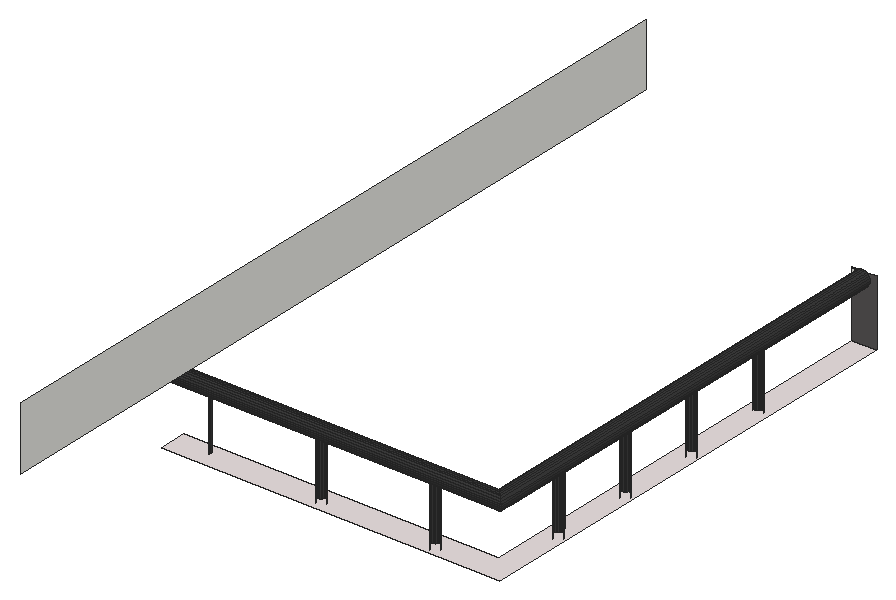
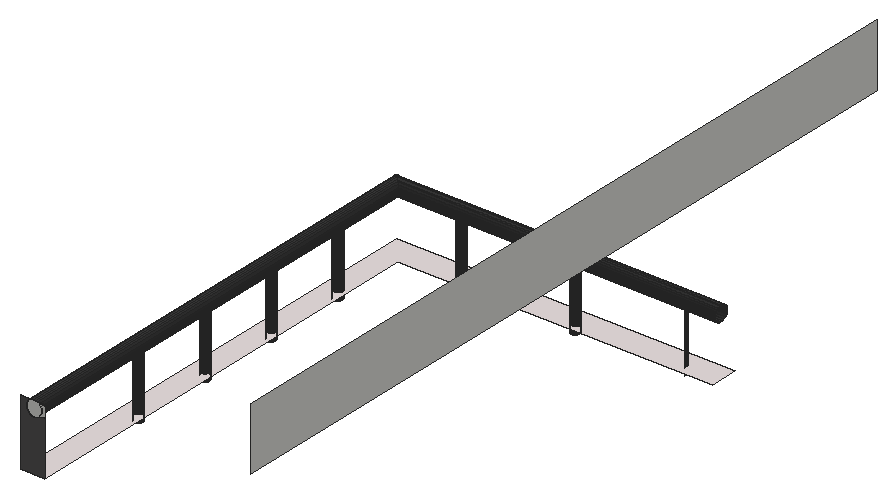
# SketchUp Ruby script. Lengths in inches.
U = 1.inch
M = Sketchup.active_model
def pt(a) = Geom::Point3d.new(a.map { |v| v * U })
def face(e, loops, mat)
  f = e.add_face(loops[0].map { |a| pt(a) })
  loops[1..].each { |l| e.add_face(l.map { |a| pt(a) }).erase! }
  f.material = f.back_material = mat if mat
  f
end
# faces: each face lists its corners as indices into pts; further lists are holes
def faces(e, pts, list, mat = nil) = list.each { |f| face(e, (f[0].is_a?(Array) ? f : [f]).map { |l| l.map { |i| pts[i] } }, mat) }
# xy, xz, yz: faces in a plane at the given z, y or x. An outline is a flat list of corners, or four numbers for a rectangle; further outlines are holes
def ring(l) = l.size == 4 ? [[l[0], l[1]], [l[2], l[1]], [l[2], l[3]], [l[0], l[3]]] : l.each_slice(2).to_a
def flat(e, list, mat, &to3) = list.each { |f| face(e, (f[0].is_a?(Array) ? f : [f]).map { |l| ring(l).map { |u, v| to3.(u, v) } }, mat) }
def xy(e, z, list, mat = nil) = flat(e, list, mat) { |x, y| [x, y, z] }
def xz(e, y, list, mat = nil) = flat(e, list, mat) { |x, z| [x, y, z] }
def yz(e, x, list, mat = nil) = flat(e, list, mat) { |y, z| [x, y, z] }
def lines(e, pts, list) = list.each { |a, b| e.add_line(pt(pts[a]), pt(pts[b])) }
# prism: a flat outline (further loops are holes) pulled along v
def prism(e, loops, v, mat = nil)
  f = face(e, loops, mat); d = Geom::Vector3d.new(v.map { |x| x * U })
  f.pushpull(f.normal.samedirection?(d) ? d.length : -d.length)
end
def box(e, o, s, mat = nil) = prism(e, [[o, [o[0] + s[0], o[1], o[2]], [o[0] + s[0], o[1] + s[1], o[2]], [o[0], o[1] + s[1], o[2]]]], [0, 0, s[2]], mat)
def at(x, y, z, deg = 0) = Geom::Transformation.translation(pt([x, y, z])) * Geom::Transformation.rotation(ORIGIN, Z_AXIS, deg.degrees)
def axes(o, x, y, z) = Geom::Transformation.new([*x, 0, *y, 0, *z, 0, *pt(o).to_a, 1])
def part(name) = M.definitions.add(name)
# library, detail: a bought-in or finely detailed component or shape, given as its bounding box
def library(name, o, s) = part(name).tap { |d| box(d.entities, o, s) }
def detail(e, o, s) = box(e.add_group.entities, o, s)
def put(e, d, t, mat = nil) = e.add_instance(d, t).tap { |i| i.material = mat if mat }
def group(e, t, mat = nil) = e.add_group.tap { |g| g.transformation = t; g.material = mat if mat }.entities
root = M.entities
M.materials.add("Generic\#2").color = [87, 84, 84]
M.materials.add("Generic\#9").color = [233, 223, 223]
M.materials.add("[Color M07]").color = [58, 58, 58]
xy(root,272.4375,[[470.29,127.4375,518.6875,127.4375,518.6875,194.75,515.25,194.75,515.25,131.45,470.29,131.45]],"Generic\#9")
xz(root,194.75,[[516.7,279.83,516.99,279.87,517.26,279.98,517.49,280.16,517.66,280.39,517.77,280.65,517.8125,280.94,517.77,281.23,517.66,281.49,517.49,281.72,517.26,281.9,516.15,281.9,515.9375,281.74,515.25,281.74,515.25,280.14,515.9375,280.14,516.15,279.98,516.42,279.87],[515.25,281.74,515.9375,281.74,516.15,281.9,515.25,281.9]])
xz(root,194.75,[[515.25,272.4375,518.6875,272.4375,518.6875,281.9,517.26,281.9,517.49,281.72,517.66,281.49,517.77,281.23,517.8125,280.94,517.77,280.65,517.66,280.39,517.49,280.16,517.26,279.98,516.99,279.87,516.7,279.83,516.42,279.87,516.15,279.98,515.9375,280.14,515.25,280.14]],"Generic\#2")
yz(root,479.73,[[90.3125,288.79,202.1875,297.79]])
p = [[490.68,129.51,271.3125],[490.83,129.45,271.3125],[490.83,129.45,280.65],[490.68,129.51,280.65],[490.99,129.43,271.3125],[490.99,129.43,280.65],
  [491.15,129.45,271.3125],[491.15,129.45,280.65],[491.3,129.51,271.3125],[491.3,129.51,280.65],[507.05,129.51,271.3125],[507.2,129.45,271.3125],
  [507.2,129.45,280.65],[507.05,129.51,280.65],[507.37,129.43,271.3125],[507.37,129.43,280.65],[507.53,129.45,271.3125],[507.53,129.45,280.65],
  [507.68,129.51,271.3125],[507.68,129.51,280.65],[490.55,129.61,271.3125],[490.55,129.61,280.65],[491.43,129.61,271.3125],[491.43,129.61,280.65],
  [506.92,129.61,271.3125],[506.92,129.61,280.65],[507.81,129.61,271.3125],[507.81,129.61,280.65],[490.45,129.74,271.3125],[490.45,129.74,280.65],
  [491.53,129.74,271.3125],[491.53,129.74,280.65],[506.82,129.74,271.3125],[506.82,129.74,280.65],[507.91,129.74,271.3125],[507.91,129.74,280.65],
  [475.16,129.74,271.3125],[475.22,129.89,271.3125],[475.22,129.89,279.83],[475.22,129.89,280.65],[475.16,129.74,280.65],[490.39,129.89,271.3125],
  [490.39,129.89,280.65],[490.39,129.89,279.83],[491.59,129.89,271.3125],[491.59,129.89,279.83],[491.59,129.89,280.65],[506.76,129.89,271.3125],
  [506.76,129.89,280.65],[506.76,129.89,279.83],[507.97,129.89,271.3125],[507.97,129.89,279.83],[507.97,129.89,280.65],[475.24,130.05,271.3125],
  [475.24,130.05,280.65],[490.37,130.05,271.3125],[490.37,130.05,280.65],[491.62,130.05,271.3125],[491.62,130.05,280.65],[506.74,130.05,271.3125],
  [506.74,130.05,280.65],[507.99,130.05,271.3125],[507.99,130.05,280.65],[475.22,130.21,271.3125],[475.22,130.21,280.65],[490.39,130.21,271.3125],
  [490.39,130.21,280.65],[491.59,130.21,271.3125],[491.59,130.21,280.65],[506.76,130.21,271.3125],[506.76,130.21,280.65],[507.97,130.21,271.3125],
  [507.97,130.21,280.65],[490.45,130.36,271.3125],[490.45,130.36,280.65],[491.53,130.36,271.3125],[491.53,130.36,280.65],[506.82,130.36,271.3125],
  [506.82,130.36,280.65],[507.91,130.36,271.3125],[507.91,130.36,280.65],[490.55,130.49,271.3125],[490.55,130.49,280.65],[491.43,130.49,271.3125],
  [491.43,130.49,280.65],[506.92,130.49,271.3125],[506.92,130.49,280.65],[507.81,130.49,271.3125],[507.81,130.49,280.65],[490.68,130.59,271.3125],
  [490.68,130.59,280.65],[491.3,130.59,271.3125],[491.3,130.59,280.65],[507.05,130.59,271.3125],[507.05,130.59,280.65],[507.68,130.59,271.3125],
  [507.68,130.59,280.65],[490.83,130.66,271.3125],[490.83,130.66,280.65],[491.15,130.66,271.3125],[491.15,130.66,280.65],[507.2,130.66,271.3125],
  [507.2,130.66,280.65],[507.53,130.66,271.3125],[507.53,130.66,280.65],[490.99,130.68,271.3125],[490.99,130.68,280.65],[507.37,130.68,271.3125],
  [507.37,130.68,280.65],[516.23,140.08,271.3125],[516.38,140.02,271.3125],[516.38,140.02,280.65],[516.23,140.08,280.65],[516.54,140,271.3125],
  [516.54,140,280.65],[516.7,140.02,271.3125],[516.7,140.02,279.83],[516.7,140.02,280.65],[516.86,140.08,271.3125],[516.86,140.08,280.65],
  [516.1,140.18,271.3125],[516.1,140.18,280.65],[516.98,140.18,271.3125],[516.98,140.18,280.65],[516,140.3125,271.3125],[516,140.3125,280.65],
  [517.08,140.3125,271.3125],[517.08,140.3125,280.65],[515.9375,140.46,271.3125],[515.9375,140.46,280.65],[517.15,140.46,271.3125],[517.15,140.46,280.65],
  [515.92,140.625,271.3125],[515.92,140.625,280.65],[517.17,140.625,271.3125],[517.17,140.625,280.65],[515.9375,140.79,271.3125],[515.9375,140.79,280.65],
  [517.15,140.79,271.3125],[517.15,140.79,280.65],[516,140.9375,271.3125],[516,140.9375,280.65],[517.08,140.9375,271.3125],[517.08,140.9375,280.65],
  [516.1,141.07,271.3125],[516.1,141.07,280.65],[516.98,141.07,271.3125],[516.98,141.07,280.65],[516.23,141.17,271.3125],[516.23,141.17,280.65],
  [516.86,141.17,271.3125],[516.86,141.17,280.65],[516.38,141.23,271.3125],[516.38,141.23,280.65],[516.54,141.25,271.3125],[516.54,141.25,280.65],
  [516.7,141.23,271.3125],[516.7,141.23,280.65],[516.7,141.23,279.83],[516.23,151.96,271.3125],[516.38,151.9,271.3125],[516.38,151.9,280.65],
  [516.23,151.96,280.65],[516.54,151.875,271.3125],[516.54,151.875,280.65],[516.7,151.9,271.3125],[516.7,151.9,279.83],[516.7,151.9,280.65],
  [516.86,151.96,271.3125],[516.86,151.96,280.65],[516.1,152.06,271.3125],[516.1,152.06,280.65],[516.98,152.06,271.3125],[516.98,152.06,280.65],
  [516,152.1875,271.3125],[516,152.1875,280.65],[517.08,152.1875,271.3125],[517.08,152.1875,280.65],[515.9375,152.34,271.3125],[515.9375,152.34,280.65],
  [517.15,152.34,271.3125],[517.15,152.34,280.65],[515.92,152.5,271.3125],[515.92,152.5,280.65],[517.17,152.5,271.3125],[517.17,152.5,280.65],
  [515.9375,152.66,271.3125],[515.9375,152.66,280.65],[517.15,152.66,271.3125],[517.15,152.66,280.65],[516,152.8125,271.3125],[516,152.8125,280.65],
  [517.08,152.8125,271.3125],[517.08,152.8125,280.65],[516.1,152.94,271.3125],[516.1,152.94,280.65],[516.98,152.94,271.3125],[516.98,152.94,280.65],
  [516.23,153.04,271.3125],[516.23,153.04,280.65],[516.86,153.04,271.3125],[516.86,153.04,280.65],[516.38,153.1,271.3125],[516.38,153.1,280.65],
  [516.7,153.1,271.3125],[516.7,153.1,279.83],[516.7,153.1,280.65],[516.54,153.125,271.3125],[516.54,153.125,280.65],[516.38,163.77,271.3125],
  [516.54,163.75,271.3125],[516.54,163.75,280.65],[516.38,163.77,280.65],[516.7,163.77,271.3125],[516.7,163.77,279.83],[516.7,163.77,280.65],
  [516.1,163.93,271.3125],[516.23,163.83,271.3125],[516.23,163.83,280.65],[516.1,163.93,280.65],[516.86,163.83,271.3125],[516.86,163.83,280.65],
  [516.98,163.93,271.3125],[516.98,163.93,280.65],[516,164.0625,271.3125],[516,164.0625,280.65],[517.08,164.0625,271.3125],[517.08,164.0625,280.65],
  [515.9375,164.21,271.3125],[515.9375,164.21,280.65],[517.15,164.21,271.3125],[517.15,164.21,280.65],[515.92,164.375,271.3125],[515.92,164.375,280.65],
  [517.17,164.375,271.3125],[517.17,164.375,280.65],[515.9375,164.54,271.3125],[515.9375,164.54,280.65],[517.15,164.54,271.3125],[517.15,164.54,280.65],
  [516,164.6875,271.3125],[516,164.6875,280.65],[517.08,164.6875,271.3125],[517.08,164.6875,280.65],[516.1,164.82,271.3125],[516.1,164.82,280.65],
  [516.98,164.82,271.3125],[516.98,164.82,280.65],[516.23,164.92,271.3125],[516.23,164.92,280.65],[516.86,164.92,271.3125],[516.86,164.92,280.65],
  [516.38,164.98,271.3125],[516.38,164.98,280.65],[516.7,164.98,271.3125],[516.7,164.98,279.83],[516.7,164.98,280.65],[516.54,165,271.3125],
  [516.54,165,280.65],[516.23,175.71,271.3125],[516.38,175.65,271.3125],[516.38,175.65,280.65],[516.23,175.71,280.65],[516.54,175.625,271.3125],
  [516.54,175.625,280.65],[516.7,175.65,271.3125],[516.7,175.65,279.83],[516.7,175.65,280.65],[516.86,175.71,271.3125],[516.86,175.71,280.65],
  [516.1,175.81,271.3125],[516.1,175.81,280.65],[516.98,175.81,271.3125],[516.98,175.81,280.65],[516,175.9375,271.3125],[516,175.9375,280.65],
  [517.08,175.9375,271.3125],[517.08,175.9375,280.65],[515.9375,176.09,271.3125],[515.9375,176.09,280.65],[517.15,176.09,271.3125],[517.15,176.09,280.65],
  [515.92,176.25,271.3125],[515.92,176.25,280.65],[517.17,176.25,271.3125],[517.17,176.25,280.65],[515.9375,176.41,271.3125],[515.9375,176.41,280.65],
  [517.15,176.41,271.3125],[517.15,176.41,280.65],[516,176.5625,271.3125],[516,176.5625,280.65],[517.08,176.5625,271.3125],[517.08,176.5625,280.65],
  [516.1,176.69,271.3125],[516.1,176.69,280.65],[516.98,176.69,271.3125],[516.98,176.69,280.65],[516.23,176.79,271.3125],[516.23,176.79,280.65],
  [516.86,176.79,271.3125],[516.86,176.79,280.65],[516.38,176.85,271.3125],[516.38,176.85,280.65],[516.7,176.85,271.3125],[516.7,176.85,279.83],
  [516.7,176.85,280.65],[516.54,176.875,271.3125],[516.54,176.875,280.65],[470.29,129.6,279.87],[470.29,129.89,279.83],[474.01,129.89,279.83],
  [516.7,129.89,279.83],[516.99,129.6,279.87],[516.7,194.75,279.83],[516.99,194.75,279.87],[516.99,131.125,279.87],[516.7,131.125,279.83],
  [470.29,130.18,279.87],[516.42,130.18,279.87],[516.42,131.125,279.87],[516.42,194.75,279.87],[470.29,129.34,279.98],[517.26,129.34,279.98],
  [517.26,194.75,279.98],[517.26,131.125,279.98],[470.29,130.44,279.98],[516.15,130.44,279.98],[516.15,131.125,279.98],[516.15,194.75,279.98],
  [470.29,129.11,280.16],[517.49,129.11,280.16],[517.49,194.75,280.16],[517.49,131.125,280.16],[470.29,130.67,280.16],[515.92,130.67,280.16],
  [515.92,131.125,280.16],[515.92,194.75,280.16],[515.9375,194.75,280.14],[470.29,128.93,280.39],[517.66,128.93,280.39],[517.66,194.75,280.39],
  [517.66,131.125,280.39],[470.29,130.85,280.39],[515.75,130.85,280.39],[515.75,131.125,280.39],[515.75,194.75,280.39],[470.29,128.82,280.65],
  [517.77,128.82,280.65],[517.77,194.75,280.65],[517.77,131.125,280.65],[470.29,130.96,280.65],[515.63,130.96,280.65],[515.63,131.125,280.65],
  [515.63,194.75,280.65],[470.29,128.78,280.94],[517.8125,128.78,280.94],[517.8125,194.75,280.94],[517.8125,131.125,280.94],[470.29,131,280.94],
  [515.6,131,280.94],[515.6,131.125,280.94],[515.6,194.75,280.94],[470.29,128.82,281.23],[517.77,128.82,281.23],[517.77,194.75,281.23],
  [517.77,131.125,281.23],[470.29,130.96,281.23],[515.63,130.96,281.23],[515.63,131.125,281.23],[515.63,194.75,281.23],[470.29,128.93,281.49],
  [517.66,128.93,281.49],[517.66,194.75,281.49],[517.66,131.125,281.49],[470.29,130.85,281.49],[515.75,130.85,281.49],[515.75,131.125,281.49],
  [515.75,194.75,281.49],[470.29,129.11,281.72],[517.49,129.11,281.72],[517.49,194.75,281.72],[517.49,131.125,281.72],[470.29,130.67,281.72],
  [515.92,130.67,281.72],[515.92,131.125,281.72],[515.92,194.75,281.72],[470.29,129.34,281.9],[517.26,129.34,281.9],[517.26,194.75,281.9],
  [517.26,131.125,281.9],[470.29,130.44,281.9],[516.15,130.44,281.9],[516.15,131.125,281.9],[516.15,194.75,281.9],[515.9375,194.75,281.74],
  [470.29,129.6,282.01],[516.99,129.6,282.01],[516.99,194.75,282.01],[516.99,131.125,282.01],[470.29,130.18,282.01],[516.42,130.18,282.01],
  [516.42,131.125,282.01],[516.42,194.75,282.01],[470.29,129.89,282.05],[516.7,129.89,282.05],[516.7,194.75,282.05],[516.7,131.125,282.05]]
faces(root,p,[[0,1,2,3],[1,4,5,2],[4,6,7,5],[6,8,9,7],[10,11,12,13],[11,14,15,12],[14,16,17,15],[16,18,19,17],
  [20,0,3,21],[8,22,23,9],[24,10,13,25],[18,26,27,19],[28,20,21,29],[22,30,31,23],[32,24,25,33],[26,34,35,27],
  [36,37,38,39,40],[41,28,29,42,43],[30,44,45,46,31],[47,32,33,48,49],[34,50,51,52,35],[37,53,54,39,38],[55,41,43,42,56],[44,57,58,46,45],
  [59,47,49,48,60],[50,61,62,52,51],[53,63,64,54],[65,55,56,66],[57,67,68,58],[69,59,60,70],[61,71,72,62],[73,65,66,74],
  [67,75,76,68],[77,69,70,78],[71,79,80,72],[81,73,74,82],[75,83,84,76],[85,77,78,86],[79,87,88,80],[89,81,82,90],
  [83,91,92,84],[93,85,86,94],[87,95,96,88],[97,89,90,98],[91,99,100,92],[101,93,94,102],[95,103,104,96],[105,97,98,106],
  [99,105,106,100],[107,101,102,108],[103,107,108,104],[109,110,111,112],[110,113,114,111],[113,115,116,117,114],[115,118,119,117,116],[120,109,112,121],
  [118,122,123,119],[124,120,121,125],[122,126,127,123],[128,124,125,129],[126,130,131,127],[132,128,129,133],[130,134,135,131],[136,132,133,137],
  [134,138,139,135],[140,136,137,141],[138,142,143,139],[144,140,141,145],[142,146,147,143],[148,144,145,149],[146,150,151,147],[152,148,149,153],
  [154,152,153,155],[156,154,155,157,158],[150,156,158,157,151],[159,160,161,162],[160,163,164,161],[163,165,166,167,164],[165,168,169,167,166],[170,159,162,171],
  [168,172,173,169],[174,170,171,175],[172,176,177,173],[178,174,175,179],[176,180,181,177],[182,178,179,183],[180,184,185,181],[186,182,183,187],
  [184,188,189,185],[190,186,187,191],[188,192,193,189],[194,190,191,195],[192,196,197,193],[198,194,195,199],[196,200,201,197],[202,198,199,203],
  [200,204,205,206,201],[207,202,203,208],[204,207,208,206,205],[209,210,211,212],[210,213,214,215,211],[216,217,218,219],[217,209,212,218],[213,220,221,215,214],
  [220,222,223,221],[224,216,219,225],[222,226,227,223],[228,224,225,229],[226,230,231,227],[232,228,229,233],[230,234,235,231],[236,232,233,237],
  [234,238,239,235],[240,236,237,241],[238,242,243,239],[244,240,241,245],[242,246,247,243],[248,244,245,249],[246,250,251,247],[252,248,249,253],
  [250,254,255,256,251],[257,252,253,258],[254,257,258,256,255],[259,260,261,262],[260,263,264,261],[263,265,266,267,264],[265,268,269,267,266],[270,259,262,271],
  [268,272,273,269],[274,270,271,275],[272,276,277,273],[278,274,275,279],[276,280,281,277],[282,278,279,283],[280,284,285,281],[286,282,283,287],
  [284,288,289,285],[290,286,287,291],[288,292,293,289],[294,290,291,295],[292,296,297,293],[298,294,295,299],[296,300,301,297],[302,298,299,303],
  [300,304,305,306,301],[307,302,303,308],[304,307,308,306,305],[309,310,311,38,43,45,49,51,312,313],[305,314,315,316,313,312,317,116,158,166,205,214,255,266],[310,318,319,312,51,49,45,43,38,311],[312,319,320,321,314,305,266,255,214,205,166,158,116,317],[322,309,313,323],
  [316,315,324,325,323,313],[318,326,327,319],[328,329,321,320,319,327],[330,322,323,331],[325,324,332,333,331,323],[326,334,335,327],[327,335,336,337,338,329,328],[339,330,331,340],
  [333,332,341,342,340,331],[334,343,344,335],[335,344,345,346,337,336],[347,339,340,348],[342,341,349,350,348,340],[343,351,352,344],[344,352,353,354,346,345],[355,347,348,356],
  [350,349,357,358,356,348],[351,359,360,352],[352,360,361,362,354,353],[363,355,356,364],[358,357,365,366,364,356],[359,367,368,360],[369,370,362,361,360,368],[371,363,364,372],
  [366,365,373,374,372,364],[367,375,376,368],[368,376,377,378,370,369],[379,371,372,380],[374,373,381,382,380,372],[375,383,384,376],[376,384,385,386,378,377],[387,379,380,388],
  [382,381,389,390,388,380],[383,391,392,384],[384,392,393,394,395,386,385],[396,387,388,397],[390,389,398,399,397,388],[391,400,401,392],[392,401,402,403,394,393],[404,396,397,405],
  [399,398,406,407,405,397],[400,404,405,401],[407,406,403,402,401,405]],"[Color M07]")
